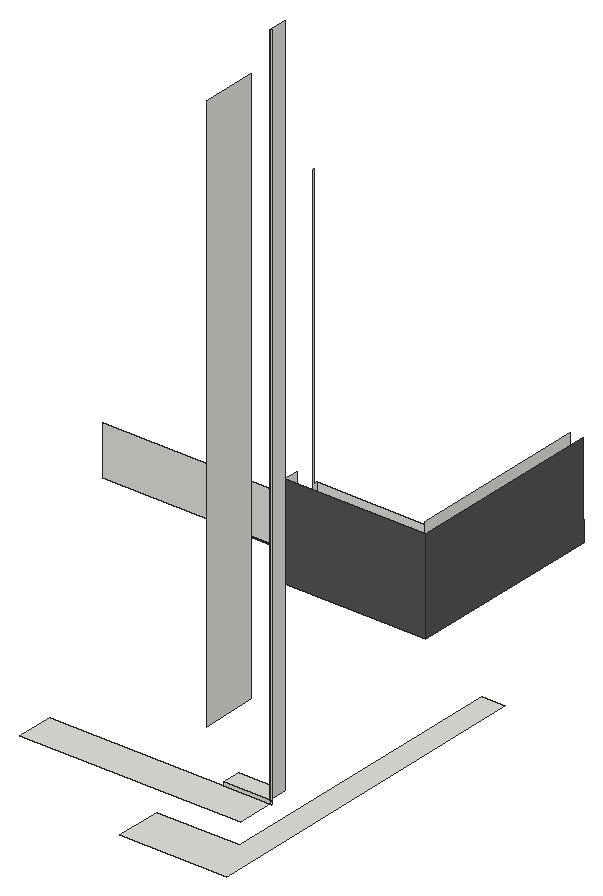
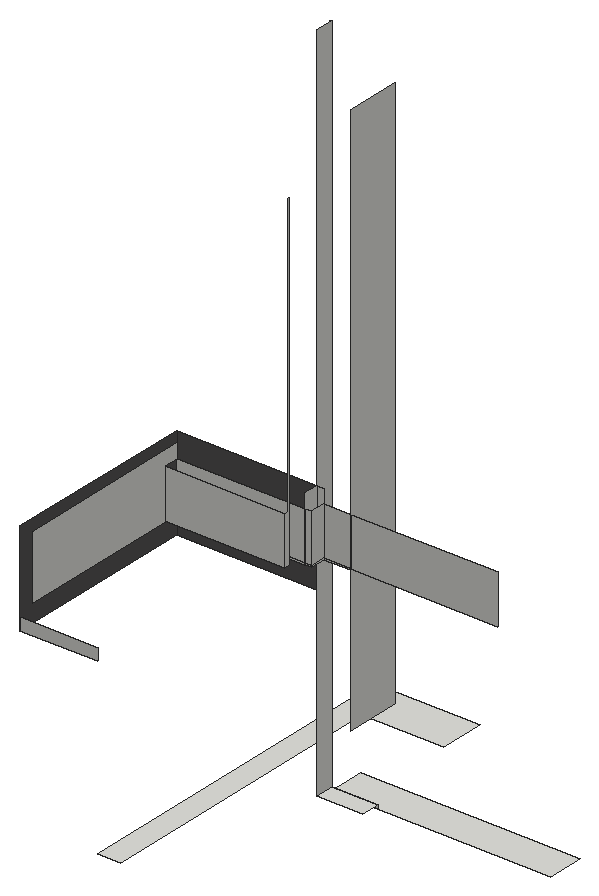
# SketchUp Ruby script. Lengths in inches.
U = 1.inch
M = Sketchup.active_model
def pt(a) = Geom::Point3d.new(a.map { |v| v * U })
def face(e, loops, mat)
  f = e.add_face(loops[0].map { |a| pt(a) })
  loops[1..].each { |l| e.add_face(l.map { |a| pt(a) }).erase! }
  f.material = f.back_material = mat if mat
  f
end
# faces: each face lists its corners as indices into pts; further lists are holes
def faces(e, pts, list, mat = nil) = list.each { |f| face(e, (f[0].is_a?(Array) ? f : [f]).map { |l| l.map { |i| pts[i] } }, mat) }
# xy, xz, yz: faces in a plane at the given z, y or x. An outline is a flat list of corners, or four numbers for a rectangle; further outlines are holes
def ring(l) = l.size == 4 ? [[l[0], l[1]], [l[2], l[1]], [l[2], l[3]], [l[0], l[3]]] : l.each_slice(2).to_a
def flat(e, list, mat, &to3) = list.each { |f| face(e, (f[0].is_a?(Array) ? f : [f]).map { |l| ring(l).map { |u, v| to3.(u, v) } }, mat) }
def xy(e, z, list, mat = nil) = flat(e, list, mat) { |x, y| [x, y, z] }
def xz(e, y, list, mat = nil) = flat(e, list, mat) { |x, z| [x, y, z] }
def yz(e, x, list, mat = nil) = flat(e, list, mat) { |y, z| [x, y, z] }
def lines(e, pts, list) = list.each { |a, b| e.add_line(pt(pts[a]), pt(pts[b])) }
# prism: a flat outline (further loops are holes) pulled along v
def prism(e, loops, v, mat = nil)
  f = face(e, loops, mat); d = Geom::Vector3d.new(v.map { |x| x * U })
  f.pushpull(f.normal.samedirection?(d) ? d.length : -d.length)
end
def box(e, o, s, mat = nil) = prism(e, [[o, [o[0] + s[0], o[1], o[2]], [o[0] + s[0], o[1] + s[1], o[2]], [o[0], o[1] + s[1], o[2]]]], [0, 0, s[2]], mat)
def at(x, y, z, deg = 0) = Geom::Transformation.translation(pt([x, y, z])) * Geom::Transformation.rotation(ORIGIN, Z_AXIS, deg.degrees)
def axes(o, x, y, z) = Geom::Transformation.new([*x, 0, *y, 0, *z, 0, *pt(o).to_a, 1])
def part(name) = M.definitions.add(name)
# library, detail: a bought-in or finely detailed component or shape, given as its bounding box
def library(name, o, s) = part(name).tap { |d| box(d.entities, o, s) }
def detail(e, o, s) = box(e.add_group.entities, o, s)
def put(e, d, t, mat = nil) = e.add_instance(d, t).tap { |i| i.material = mat if mat }
def group(e, t, mat = nil) = e.add_group.tap { |g| g.transformation = t; g.material = mat if mat }.entities
root = M.entities
M.materials.add("Generic\#2").color = [87, 84, 84]
xy(root,51,[[394.85,108.375,470.29,120.9375]])
xy(root,52.25,[[454.48,120.9375,470.29,127.4375]])
xy(root,56.4375,[[455.52,75.375,491.875,75.375,491.875,194.8125,483.89,194.8125,483.89,90.9375,455.52,90.9375]])
xy(root,126,[[467.91,127.4375,470.29,132.5625]])
xz(root,120.9375,[[454.48,51,470.29,52.25],[470.29,51,470.85,52.25],[470.29,52.25,470.85,288.79]])
xz(root,127.4375,[[458.64,126,467.91,126.47],[467.91,126,470.29,148.0625],[407.84,126.47,458.64,143.28],[458.64,126.47,467.91,143.28]])
xz(root,127.4375,[[470.29,115.8125,518.6875,148.0625]],"Generic\#2")
xz(root,132.5625,[[467.91,126,470.29,126.47],[470.29,126,514.25,126.47],[467.91,126.47,470.29,143.28],[470.29,126.47,514.25,143.28]])
xz(root,138,[[472.76,126.47,514.25,143.28]])
xz(root,194.8125,[[491.875,115.8125,518.6875,120]])
yz(root,458.64,[[108.375,76.26,127.4375,268.37]])
yz(root,467.91,[[127.4375,126,132.5625,126.47],[127.4375,126.47,132.5625,143.28]])
yz(root,470.29,[[120.9375,52.25,127.4375,288.79],[127.4375,126,132.5625,148.0625]])
yz(root,472.76,[[136.1875,126.47,136.1875,240,136.78,240,136.78,143.28,138,143.28,138,126.47]])
yz(root,514.25,[[132.5625,126,132.5625,126.47,138,126.47,138,143.28,132.5625,143.28,132.5625,148.0625,194.75,148.0625,194.75,126]])
yz(root,518.6875,[[127.4375,115.8125,194.8125,115.8125,194.8125,120,194.75,126,194.75,148.0625,127.4375,148.0625]],"Generic\#2")
